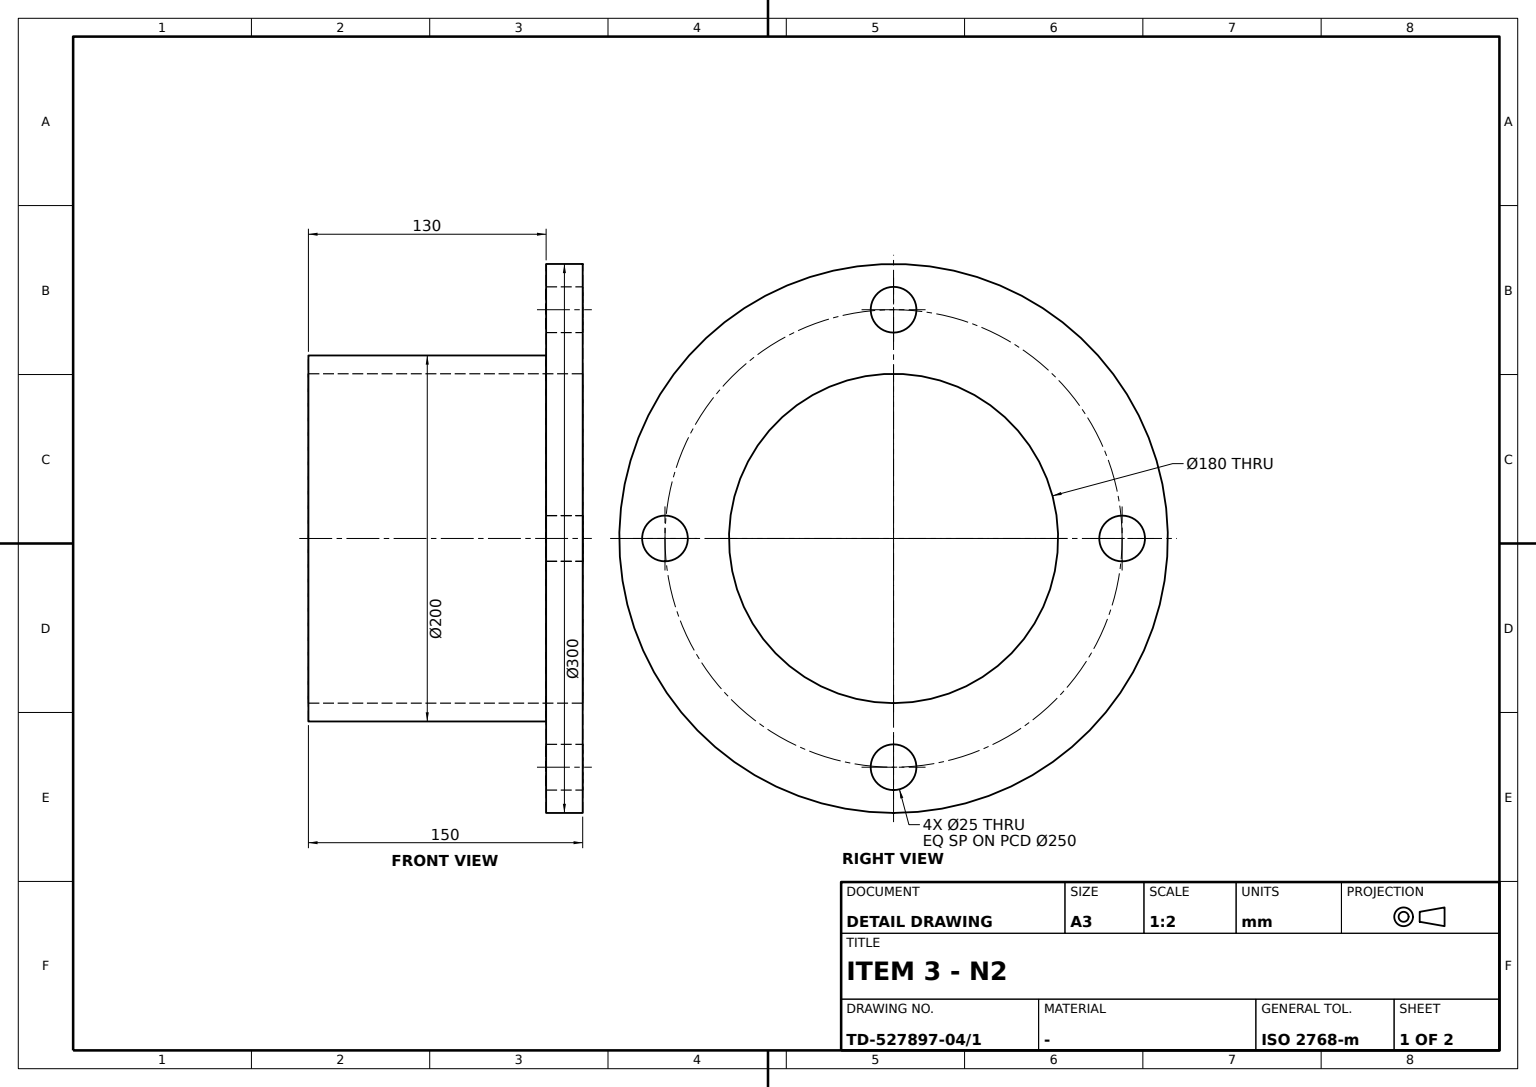
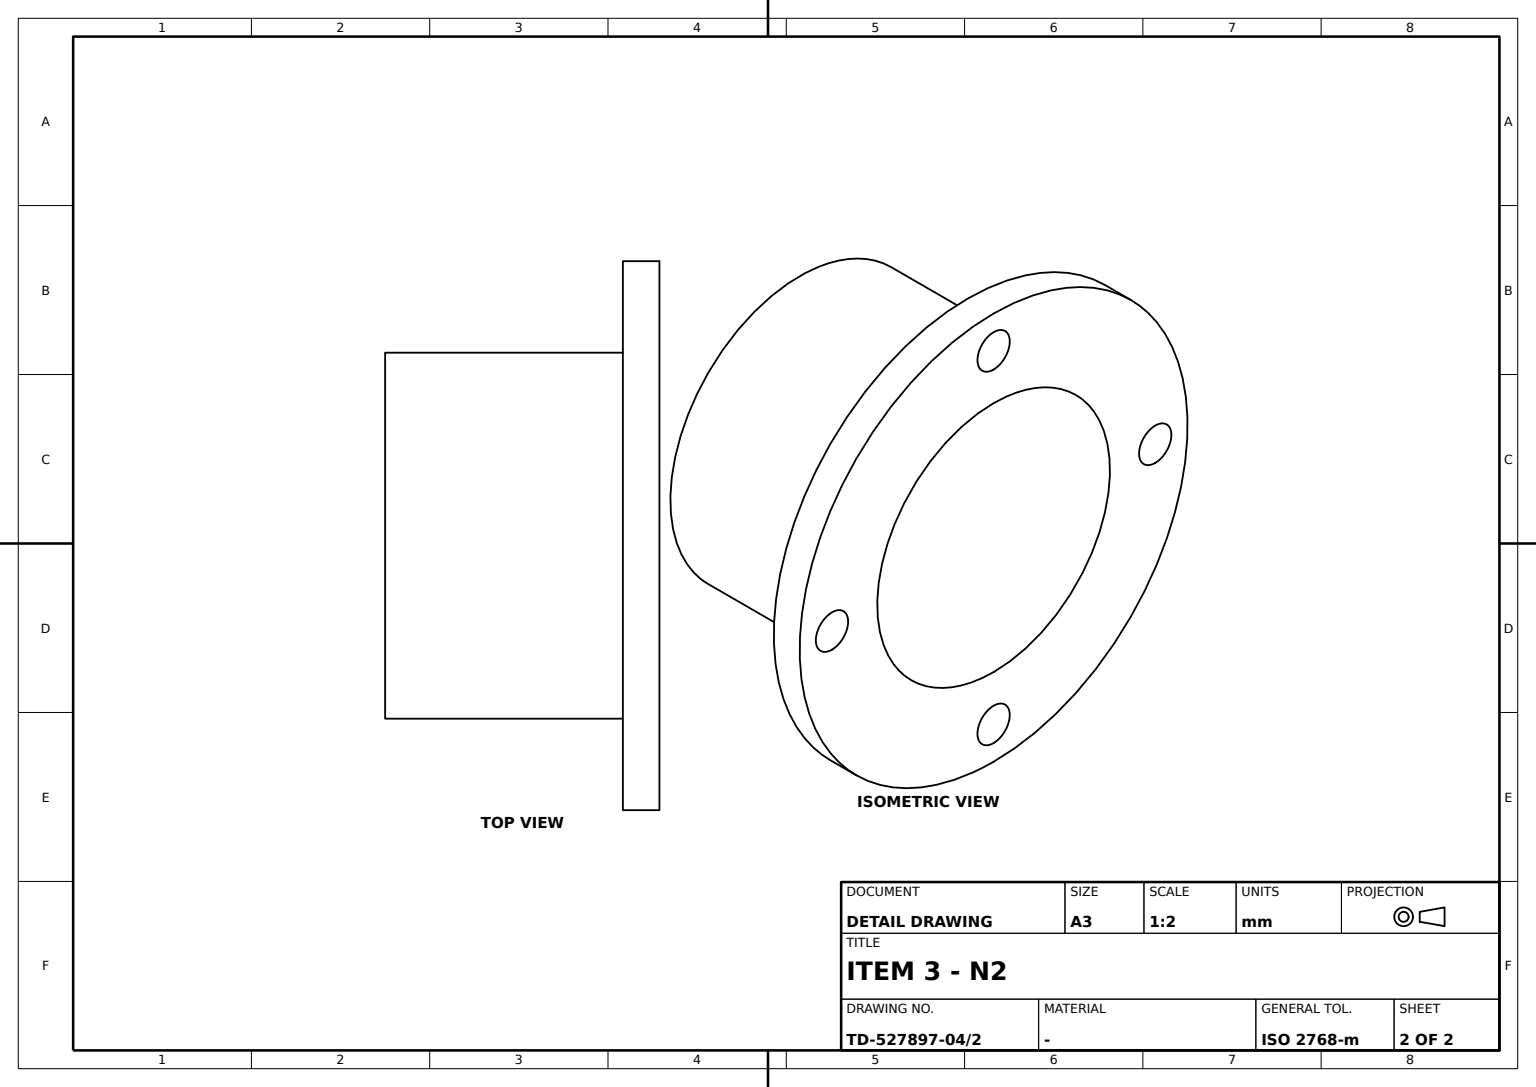
ISO-10303-21;
HEADER;
FILE_DESCRIPTION((''),'2;1');
FILE_NAME('','',(''),(''),'','','');
FILE_SCHEMA(('AUTOMOTIVE_DESIGN'));
ENDSEC;
DATA;
#1=APPLICATION_CONTEXT('');
#2=PRODUCT_CONTEXT('',#1,'mechanical');
#3=PRODUCT('','','',(#2));
#4=PRODUCT_DEFINITION_FORMATION('','',#3);
#5=PRODUCT_DEFINITION_CONTEXT('',#1,'design');
#6=PRODUCT_DEFINITION('','',#4,#5);
#7=PRODUCT_DEFINITION_SHAPE('','',#6);
#8=(LENGTH_UNIT()NAMED_UNIT(*)SI_UNIT(.MILLI.,.METRE.));
#9=(NAMED_UNIT(*)PLANE_ANGLE_UNIT()SI_UNIT($,.RADIAN.));
#10=(NAMED_UNIT(*)SI_UNIT($,.STERADIAN.)SOLID_ANGLE_UNIT());
#11=UNCERTAINTY_MEASURE_WITH_UNIT(LENGTH_MEASURE(0.005),#8,'distance_accuracy_value','');
#12=(GEOMETRIC_REPRESENTATION_CONTEXT(3)GLOBAL_UNCERTAINTY_ASSIGNED_CONTEXT((#11))GLOBAL_UNIT_ASSIGNED_CONTEXT((#8,#9,#10))REPRESENTATION_CONTEXT('',''));
#13=CARTESIAN_POINT('',(-1137.509741,-1275.,2630.));
#14=VERTEX_POINT('',#13);
#15=CARTESIAN_POINT('',(-1150.009741,-1275.,2630.));
#16=DIRECTION('',(0.,0.,1.));
#17=DIRECTION('',(1.,0.,0.));
#18=AXIS2_PLACEMENT_3D('',#15,#16,#17);
#19=CIRCLE('',#18,12.5);
#20=EDGE_CURVE('',#14,#14,#19,.T.);
#21=ORIENTED_EDGE('',*,*,#20,.F.);
#22=EDGE_LOOP('',(#21));
#23=FACE_BOUND('',#22,.T.);
#24=CARTESIAN_POINT('',(-1137.509741,-1275.,2650.));
#25=VERTEX_POINT('',#24);
#26=CARTESIAN_POINT('',(-1150.009741,-1275.,2650.));
#27=AXIS2_PLACEMENT_3D('',#26,#16,#17);
#28=CIRCLE('',#27,12.5);
#29=EDGE_CURVE('',#25,#25,#28,.T.);
#30=ORIENTED_EDGE('',*,*,#29,.T.);
#31=EDGE_LOOP('',(#30));
#32=FACE_BOUND('',#31,.T.);
#33=CARTESIAN_POINT('',(-1150.009741,-1275.,2640.));
#34=AXIS2_PLACEMENT_3D('',#33,#16,#17);
#35=CYLINDRICAL_SURFACE('',#34,12.5);
#36=ADVANCED_FACE('',(#23,#32),#35,.F.);
#37=CARTESIAN_POINT('',(-1050.,-1150.,2500.));
#38=VERTEX_POINT('',#37);
#39=CARTESIAN_POINT('',(-1150.,-1150.,2500.));
#40=AXIS2_PLACEMENT_3D('',#39,#16,#17);
#41=CIRCLE('',#40,100.);
#42=EDGE_CURVE('',#38,#38,#41,.T.);
#43=ORIENTED_EDGE('',*,*,#42,.T.);
#44=EDGE_LOOP('',(#43));
#45=FACE_BOUND('',#44,.T.);
#46=CARTESIAN_POINT('',(-1050.,-1150.,2630.));
#47=VERTEX_POINT('',#46);
#48=CARTESIAN_POINT('',(-1150.,-1150.,2630.));
#49=AXIS2_PLACEMENT_3D('',#48,#16,#17);
#50=CIRCLE('',#49,100.);
#51=EDGE_CURVE('',#47,#47,#50,.T.);
#52=ORIENTED_EDGE('',*,*,#51,.F.);
#53=EDGE_LOOP('',(#52));
#54=FACE_BOUND('',#53,.T.);
#55=CARTESIAN_POINT('',(-1150.,-1150.,2640.));
#56=AXIS2_PLACEMENT_3D('',#55,#16,#17);
#57=CYLINDRICAL_SURFACE('',#56,100.);
#58=ADVANCED_FACE('',(#45,#54),#57,.T.);
#59=CARTESIAN_POINT('',(-1262.5,-1149.990259,2630.));
#60=VERTEX_POINT('',#59);
#61=CARTESIAN_POINT('',(-1275.,-1149.990259,2630.));
#62=AXIS2_PLACEMENT_3D('',#61,#16,#17);
#63=CIRCLE('',#62,12.5);
#64=EDGE_CURVE('',#60,#60,#63,.T.);
#65=ORIENTED_EDGE('',*,*,#64,.T.);
#66=EDGE_LOOP('',(#65));
#67=FACE_BOUND('',#66,.T.);
#68=ORIENTED_EDGE('',*,*,#20,.T.);
#69=EDGE_LOOP('',(#68));
#70=FACE_BOUND('',#69,.T.);
#71=CARTESIAN_POINT('',(-1137.490259,-1025.,2630.));
#72=VERTEX_POINT('',#71);
#73=CARTESIAN_POINT('',(-1149.990259,-1025.,2630.));
#74=AXIS2_PLACEMENT_3D('',#73,#16,#17);
#75=CIRCLE('',#74,12.5);
#76=EDGE_CURVE('',#72,#72,#75,.T.);
#77=ORIENTED_EDGE('',*,*,#76,.T.);
#78=EDGE_LOOP('',(#77));
#79=FACE_BOUND('',#78,.T.);
#80=CARTESIAN_POINT('',(-1012.5,-1150.009741,2630.));
#81=VERTEX_POINT('',#80);
#82=CARTESIAN_POINT('',(-1025.,-1150.009741,2630.));
#83=AXIS2_PLACEMENT_3D('',#82,#16,#17);
#84=CIRCLE('',#83,12.5);
#85=EDGE_CURVE('',#81,#81,#84,.T.);
#86=ORIENTED_EDGE('',*,*,#85,.T.);
#87=EDGE_LOOP('',(#86));
#88=FACE_BOUND('',#87,.T.);
#89=CARTESIAN_POINT('',(-1000.,-1150.,2630.));
#90=VERTEX_POINT('',#89);
#91=CIRCLE('',#49,150.);
#92=EDGE_CURVE('',#90,#90,#91,.T.);
#93=ORIENTED_EDGE('',*,*,#92,.F.);
#94=EDGE_LOOP('',(#93));
#95=FACE_BOUND('',#94,.T.);
#96=ORIENTED_EDGE('',*,*,#51,.T.);
#97=EDGE_LOOP('',(#96));
#98=FACE_BOUND('',#97,.T.);
#99=CARTESIAN_POINT('',(0.,0.,2630.));
#100=AXIS2_PLACEMENT_3D('',#99,#16,#17);
#101=PLANE('',#100);
#102=ADVANCED_FACE('',(#67,#70,#79,#88,#95,#98),#101,.F.);
#103=CARTESIAN_POINT('',(-1012.5,-1150.009741,2650.));
#104=VERTEX_POINT('',#103);
#105=CARTESIAN_POINT('',(-1025.,-1150.009741,2650.));
#106=AXIS2_PLACEMENT_3D('',#105,#16,#17);
#107=CIRCLE('',#106,12.5);
#108=EDGE_CURVE('',#104,#104,#107,.T.);
#109=ORIENTED_EDGE('',*,*,#108,.F.);
#110=EDGE_LOOP('',(#109));
#111=FACE_BOUND('',#110,.T.);
#112=CARTESIAN_POINT('',(-1060.,-1150.,2650.));
#113=VERTEX_POINT('',#112);
#114=CARTESIAN_POINT('',(-1150.,-1150.,2650.));
#115=AXIS2_PLACEMENT_3D('',#114,#16,#17);
#116=CIRCLE('',#115,90.);
#117=EDGE_CURVE('',#113,#113,#116,.T.);
#118=ORIENTED_EDGE('',*,*,#117,.F.);
#119=EDGE_LOOP('',(#118));
#120=FACE_BOUND('',#119,.T.);
#121=CARTESIAN_POINT('',(-1137.490259,-1025.,2650.));
#122=VERTEX_POINT('',#121);
#123=CARTESIAN_POINT('',(-1149.990259,-1025.,2650.));
#124=AXIS2_PLACEMENT_3D('',#123,#16,#17);
#125=CIRCLE('',#124,12.5);
#126=EDGE_CURVE('',#122,#122,#125,.T.);
#127=ORIENTED_EDGE('',*,*,#126,.F.);
#128=EDGE_LOOP('',(#127));
#129=FACE_BOUND('',#128,.T.);
#130=CARTESIAN_POINT('',(-1262.5,-1149.990259,2650.));
#131=VERTEX_POINT('',#130);
#132=CARTESIAN_POINT('',(-1275.,-1149.990259,2650.));
#133=AXIS2_PLACEMENT_3D('',#132,#16,#17);
#134=CIRCLE('',#133,12.5);
#135=EDGE_CURVE('',#131,#131,#134,.T.);
#136=ORIENTED_EDGE('',*,*,#135,.F.);
#137=EDGE_LOOP('',(#136));
#138=FACE_BOUND('',#137,.T.);
#139=CARTESIAN_POINT('',(-1000.,-1150.,2650.));
#140=VERTEX_POINT('',#139);
#141=CIRCLE('',#115,150.);
#142=EDGE_CURVE('',#140,#140,#141,.T.);
#143=ORIENTED_EDGE('',*,*,#142,.T.);
#144=EDGE_LOOP('',(#143));
#145=FACE_BOUND('',#144,.T.);
#146=ORIENTED_EDGE('',*,*,#29,.F.);
#147=EDGE_LOOP('',(#146));
#148=FACE_BOUND('',#147,.T.);
#149=CARTESIAN_POINT('',(0.,0.,2650.));
#150=AXIS2_PLACEMENT_3D('',#149,#16,#17);
#151=PLANE('',#150);
#152=ADVANCED_FACE('',(#111,#120,#129,#138,#145,#148),#151,.T.);
#153=ORIENTED_EDGE('',*,*,#64,.F.);
#154=EDGE_LOOP('',(#153));
#155=FACE_BOUND('',#154,.T.);
#156=ORIENTED_EDGE('',*,*,#135,.T.);
#157=EDGE_LOOP('',(#156));
#158=FACE_BOUND('',#157,.T.);
#159=CARTESIAN_POINT('',(-1275.,-1149.990259,2640.));
#160=AXIS2_PLACEMENT_3D('',#159,#16,#17);
#161=CYLINDRICAL_SURFACE('',#160,12.5);
#162=ADVANCED_FACE('',(#155,#158),#161,.F.);
#163=ORIENTED_EDGE('',*,*,#85,.F.);
#164=EDGE_LOOP('',(#163));
#165=FACE_BOUND('',#164,.T.);
#166=ORIENTED_EDGE('',*,*,#108,.T.);
#167=EDGE_LOOP('',(#166));
#168=FACE_BOUND('',#167,.T.);
#169=CARTESIAN_POINT('',(-1025.,-1150.009741,2640.));
#170=AXIS2_PLACEMENT_3D('',#169,#16,#17);
#171=CYLINDRICAL_SURFACE('',#170,12.5);
#172=ADVANCED_FACE('',(#165,#168),#171,.F.);
#173=ORIENTED_EDGE('',*,*,#42,.F.);
#174=EDGE_LOOP('',(#173));
#175=FACE_BOUND('',#174,.T.);
#176=CARTESIAN_POINT('',(-1060.,-1150.,2500.));
#177=VERTEX_POINT('',#176);
#178=CIRCLE('',#40,90.);
#179=EDGE_CURVE('',#177,#177,#178,.T.);
#180=ORIENTED_EDGE('',*,*,#179,.T.);
#181=EDGE_LOOP('',(#180));
#182=FACE_BOUND('',#181,.T.);
#183=CARTESIAN_POINT('',(0.,0.,2500.));
#184=AXIS2_PLACEMENT_3D('',#183,#16,#17);
#185=PLANE('',#184);
#186=ADVANCED_FACE('',(#175,#182),#185,.F.);
#187=ORIENTED_EDGE('',*,*,#76,.F.);
#188=EDGE_LOOP('',(#187));
#189=FACE_BOUND('',#188,.T.);
#190=ORIENTED_EDGE('',*,*,#126,.T.);
#191=EDGE_LOOP('',(#190));
#192=FACE_BOUND('',#191,.T.);
#193=CARTESIAN_POINT('',(-1149.990259,-1025.,2640.));
#194=AXIS2_PLACEMENT_3D('',#193,#16,#17);
#195=CYLINDRICAL_SURFACE('',#194,12.5);
#196=ADVANCED_FACE('',(#189,#192),#195,.F.);
#197=ORIENTED_EDGE('',*,*,#142,.F.);
#198=EDGE_LOOP('',(#197));
#199=FACE_BOUND('',#198,.T.);
#200=ORIENTED_EDGE('',*,*,#92,.T.);
#201=EDGE_LOOP('',(#200));
#202=FACE_BOUND('',#201,.T.);
#203=CYLINDRICAL_SURFACE('',#56,150.);
#204=ADVANCED_FACE('',(#199,#202),#203,.T.);
#205=ORIENTED_EDGE('',*,*,#117,.T.);
#206=EDGE_LOOP('',(#205));
#207=FACE_BOUND('',#206,.T.);
#208=ORIENTED_EDGE('',*,*,#179,.F.);
#209=EDGE_LOOP('',(#208));
#210=FACE_BOUND('',#209,.T.);
#211=CARTESIAN_POINT('',(-1150.,-1150.,2575.));
#212=AXIS2_PLACEMENT_3D('',#211,#16,#17);
#213=CYLINDRICAL_SURFACE('',#212,90.);
#214=ADVANCED_FACE('',(#207,#210),#213,.F.);
#215=CLOSED_SHELL('',(#36,#58,#102,#152,#162,#172,#186,#196,#204,#214));
#216=MANIFOLD_SOLID_BREP('',#215);
#217=ADVANCED_BREP_SHAPE_REPRESENTATION('',(#216),#12);
#218=SHAPE_DEFINITION_REPRESENTATION(#7,#217);
ENDSEC;
END-ISO-10303-21;
